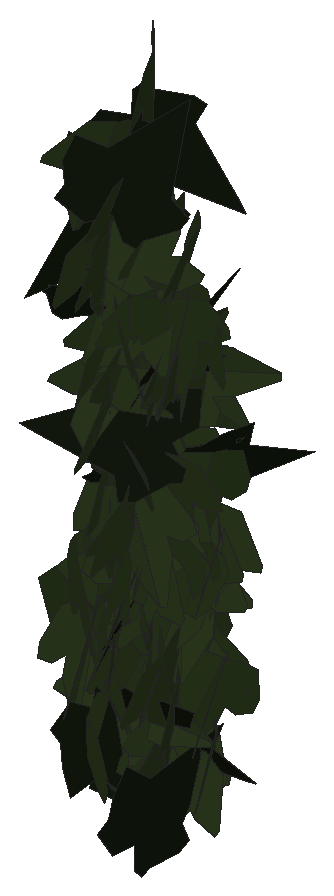
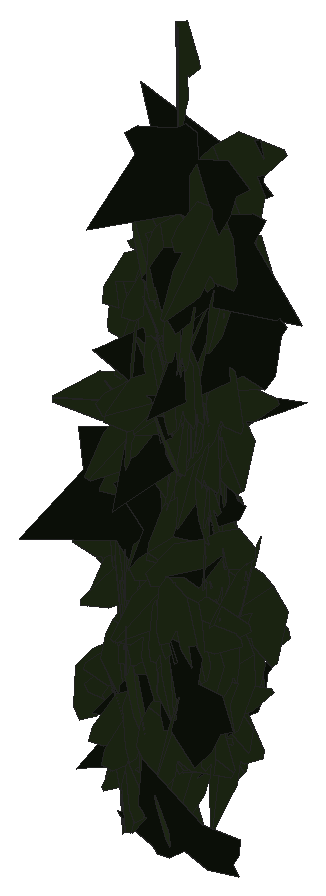
# SketchUp Ruby script. Lengths in inches.
U = 1.inch
M = Sketchup.active_model
def pt(a) = Geom::Point3d.new(a.map { |v| v * U })
def face(e, loops, mat)
  f = e.add_face(loops[0].map { |a| pt(a) })
  loops[1..].each { |l| e.add_face(l.map { |a| pt(a) }).erase! }
  f.material = f.back_material = mat if mat
  f
end
# faces: each face lists its corners as indices into pts; further lists are holes
def faces(e, pts, list, mat = nil) = list.each { |f| face(e, (f[0].is_a?(Array) ? f : [f]).map { |l| l.map { |i| pts[i] } }, mat) }
# xy, xz, yz: faces in a plane at the given z, y or x. An outline is a flat list of corners, or four numbers for a rectangle; further outlines are holes
def ring(l) = l.size == 4 ? [[l[0], l[1]], [l[2], l[1]], [l[2], l[3]], [l[0], l[3]]] : l.each_slice(2).to_a
def flat(e, list, mat, &to3) = list.each { |f| face(e, (f[0].is_a?(Array) ? f : [f]).map { |l| ring(l).map { |u, v| to3.(u, v) } }, mat) }
def xy(e, z, list, mat = nil) = flat(e, list, mat) { |x, y| [x, y, z] }
def xz(e, y, list, mat = nil) = flat(e, list, mat) { |x, z| [x, y, z] }
def yz(e, x, list, mat = nil) = flat(e, list, mat) { |y, z| [x, y, z] }
def lines(e, pts, list) = list.each { |a, b| e.add_line(pt(pts[a]), pt(pts[b])) }
# prism: a flat outline (further loops are holes) pulled along v
def prism(e, loops, v, mat = nil)
  f = face(e, loops, mat); d = Geom::Vector3d.new(v.map { |x| x * U })
  f.pushpull(f.normal.samedirection?(d) ? d.length : -d.length)
end
def box(e, o, s, mat = nil) = prism(e, [[o, [o[0] + s[0], o[1], o[2]], [o[0] + s[0], o[1] + s[1], o[2]], [o[0], o[1] + s[1], o[2]]]], [0, 0, s[2]], mat)
def at(x, y, z, deg = 0) = Geom::Transformation.translation(pt([x, y, z])) * Geom::Transformation.rotation(ORIGIN, Z_AXIS, deg.degrees)
def axes(o, x, y, z) = Geom::Transformation.new([*x, 0, *y, 0, *z, 0, *pt(o).to_a, 1])
def part(name) = M.definitions.add(name)
# library, detail: a bought-in or finely detailed component or shape, given as its bounding box
def library(name, o, s) = part(name).tap { |d| box(d.entities, o, s) }
def detail(e, o, s) = box(e.add_group.entities, o, s)
def put(e, d, t, mat = nil) = e.add_instance(d, t).tap { |i| i.material = mat if mat }
def group(e, t, mat = nil) = e.add_group.tap { |g| g.transformation = t; g.material = mat if mat }.entities
root = M.entities
M.materials.add("efeu1").color = [18, 25, 13]
M.materials.add("efeu2").color = [43, 57, 29]
c1 = part("ivyleaf_10")
p = [[0,0.5,-0.03],[-0.0625,2.02,-0.43],[-0.19,2.01,-0.46],[-0.54,1.05,-0.29],[-0.52,0.625,-0.18],[-0.83,0.76,-0.28],
  [-1.16,0.64,-0.33],[-1.15,0.33,-0.24],[-0.77,-0.39,0.02],[-0.3,-0.51,0.16],[0.04,-0.48,0.23],[-0.02,2.01,-0.4375],
  [-0.06,2.01,-0.43],[0.04,-0.49,0.23],[0.67,-0.49,0.14],[1.38,0.36,-0.2],[1.375,0.51,-0.24],[0.81,0.65,-0.19],
  [0.62,0.59,-0.15],[0.6,1.09,-0.28],[0.5,1.23,-0.31]]
faces(c1.entities,p,[[0,1,2,3,4,5,6,7,8,9,10],[11,12,0,13,14,15,16,17,18,19,20]],"efeu2")
c2 = part("ivyleaf_9")
p = [[1.54,2.16,1.25],[1.36,2.04,1.19],[-0.21,0.99,0.68],[-0.71,1.11,0.82],[-0.85,0.86,0.67],[-0.8,0.17,0.21],
  [-0.9,-0.01,0.1],[-0.67,-0.16,-0.02],[-0.08,-0.08,-0.05],[-0.03,-0.6,-0.4],[0.65,-0.88,-0.66],[0.83,-0.6,-0.49],
  [1.29,-0.42,-0.43],[1.8125,-0.07,-0.26],[1.21,0.44,0.15]]
faces(c2.entities,p,[[0,1,2,3,4,5,6,7,8,9,10,11,12,13,14]],"efeu1")
put(root,c1,axes([22.6875,224.7,214.85],[0.03755,-0.45322,-0.20781],[0.02712,0.20995,-0.45298],[0.49785,0.02275,0.04035]))
put(root,c1,axes([22.68,225.04,220.85],[-0.06561,-0.31766,-0.38051],[0.06416,0.37516,-0.32425],[0.49151,-0.09137,-0.00847]))
put(root,c1,axes([22.625,224.47,216.64],[-0.12805,0.47925,-0.06261],[0.01255,-0.06145,-0.49605],[-0.48316,-0.12861,0.00371]))
put(root,c1,axes([22.62,225.15,217.17],[0.2593,0.42528,-0.04357],[-0.02338,-0.03677,-0.4981],[-0.42687,0.26035,0.00082]))
put(root,c2,axes([22.86,224.98,220.58],[-0.04237,0.13988,-0.47816],[-0.02365,-0.47991,-0.1383],[-0.49764,0.01089,0.04728]))
put(root,c1,axes([22.73,224.58,215.93],[-0.17611,0.39993,-0.24299],[-0.09749,-0.28528,-0.39889],[-0.45769,-0.09312,0.17846]))
put(root,c1,axes([22.8125,224.86,218.66],[-0.27515,-0.37614,0.18114],[-0.04696,-0.18768,-0.46105],[0.41483,-0.27073,0.06795]))
put(root,c2,axes([22.71,225.38,213.77],[-0.41978,0.11401,0.24655],[0.23878,-0.06145,0.43498],[0.12949,0.48293,-0.00285]))
put(root,c1,axes([22.78,225.24,216.72],[-0.05871,-0.49513,0.03748],[-0.00529,-0.03711,-0.49859],[0.49651,-0.05894,-0.00088]))
put(root,c1,axes([22.86,225.27,216.29],[-0.36011,-0.31008,0.15546],[-0.09856,-0.12339,-0.47441],[0.33258,-0.37232,0.02774]))
put(root,c1,axes([22.78,224.65,221.42],[-0.12903,-0.4572,0.15595],[-0.00367,-0.16049,-0.47353],[0.48305,-0.12335,0.03806]))
put(root,c2,axes([22.57,224.55,219.71],[0.41909,0.25918,0.0848],[0.06905,0.04955,-0.49272],[-0.26381,0.4247,0.00574]))
put(root,c1,axes([22.77,224.91,219.05],[-0.48868,0.10307,-0.02389],[0.02379,-0.00294,-0.49942],[-0.10309,-0.48925,-0.00203]))
put(root,c1,axes([22.79,224.9,215.09],[-0.2091,-0.37415,0.25747],[0.05261,-0.30149,-0.39539],[0.45112,-0.13826,0.16545]))
put(root,c1,axes([22.75,224.46,220.32],[-0.01591,-0.43719,-0.2421],[0.08308,0.23653,-0.43261],[0.49279,-0.05399,0.06511]))
put(root,c1,axes([22.72,224.55,215.9],[0.30488,0.3849,-0.09434],[-0.05987,-0.07292,-0.49102],[-0.39175,0.31069,0.00163]))
put(root,c1,axes([22.89,225.42,215.2],[-0.0647,-0.34983,0.35133],[-0.08214,-0.34185,-0.35551],[0.48894,-0.10372,-0.01323]))
put(root,c1,axes([22.55,224.45,216.36],[-0.36033,-0.01903,-0.34612],[0.34663,-0.01684,-0.35995],[0.00204,-0.49935,0.02533]))
put(root,c1,axes([22.8,224.73,217.67],[0.14279,-0.42704,-0.21736],[0.01533,0.23076,-0.4433],[0.47893,0.11994,0.07899]))
put(root,c1,axes([22.61,225.16,217.99],[0.10332,-0.27071,0.40748],[0.28349,-0.30628,-0.27537],[0.39869,0.28794,0.0902]))
put(root,c1,axes([22.91,225.31,216.3],[-0.38221,-0.32073,0.03236],[-0.01778,-0.02913,-0.49883],[0.32187,-0.38247,0.01086]))
put(root,c1,axes([22.85,225,218.37],[-0.45896,0.19836,-0.0037],[0.00135,-0.00622,-0.49996],[-0.19839,-0.45893,0.00518]))
put(root,c1,axes([22.86,224.57,219.16],[0.02583,-0.40557,-0.29129],[0.02986,0.29241,-0.40448],[0.49844,0.0035,0.03932]))
put(root,c1,axes([22.92,224.83,217.88],[0.31506,-0.35458,-0.15814],[-0.10861,0.11504,-0.47431],[0.37275,0.33323,-0.00454]))
put(root,c1,axes([22.62,224.59,215.66],[-0.27958,0.21403,-0.355],[0.28131,-0.21653,-0.3521],[-0.30446,-0.39662,0.00066]))
put(root,c1,axes([22.8,225.1,219.28],[0.3207,-0.38339,0.01257],[0.1001,0.06782,-0.48516],[0.37031,0.3137,0.12026]))
put(root,c1,axes([22.9375,224.45,218.49],[0.13648,-0.45371,-0.15976],[-0.02047,0.16044,-0.47312],[0.48058,0.13569,0.02522]))
put(root,c1,axes([22.95,224.83,219.25],[-0.41607,-0.27599,-0.02676],[0.02157,0.0159,-0.49928],[0.27644,-0.41663,-0.00132]))
put(root,c1,axes([22.9375,225.01,217.37],[-0.13005,-0.46452,-0.13155],[0.04299,0.12455,-0.48233],[0.48087,-0.13676,0.00754]))
put(root,c2,axes([22.56,225.4,215.74],[0.01543,-0.0039,-0.49975],[0.41582,0.27746,0.01067],[0.27724,-0.41593,0.01181]))
put(root,c1,axes([23.14,224.52,218.03],[-0.37486,0.17021,0.28374],[-0.27494,0.07832,-0.41021],[-0.18409,-0.46357,0.03488]))
put(root,c1,axes([22.98,225.26,216.34],[0.05158,-0.4815,-0.12451],[-0.00997,0.12415,-0.48424],[0.49723,0.05244,0.0032]))
put(root,c1,axes([22.97,224.37,220.4],[0.16693,-0.45223,-0.13276],[0.00027,0.14093,-0.47973],[0.47131,0.16009,0.0473]))
put(root,c1,axes([23,224.49,216.09],[0.26145,-0.33283,-0.26621],[-0.0576,0.28185,-0.40895],[0.42228,0.24451,0.10904]))
put(root,c1,axes([22.85,225.01,214.62],[0.19151,0.45262,0.09197],[0.03571,0.08476,-0.49147],[-0.46049,0.19481,0.00014]))
put(root,c1,axes([23,225.28,216.5],[-0.25697,-0.42425,-0.06308],[0.03797,0.05074,-0.49597],[0.42723,-0.25969,0.00614]))
put(root,c1,axes([22.84,225.23,216.95],[-0.15281,-0.30265,-0.36749],[0.25408,0.27455,-0.33176],[0.40261,-0.28814,0.06988]))
put(root,c1,axes([23.07,224.18,214.92],[-0.17796,0.40184,0.23843],[-0.11876,0.20787,-0.43896],[-0.45191,-0.21287,0.02146]))
put(root,c1,axes([23.05,225.04,216.46],[0.04266,-0.48287,0.12254],[0.01746,-0.12146,-0.48471],[0.49787,0.04563,0.00649]))
put(root,c1,axes([22.99,224.6,218.94],[0.19174,-0.4321,0.16286],[0.07881,-0.14313,-0.47255],[0.455,0.20688,0.01322]))
put(root,c1,axes([23.05,224.47,220.99],[0.1837,-0.46417,0.02829],[0.00395,-0.02886,-0.49915],[0.46501,0.18361,-0.00694]))
put(root,c1,axes([22.93,225.26,215.32],[-0.17641,0.35657,-0.30288],[0.08652,-0.29325,-0.39563],[-0.45977,-0.192,0.04176]))
put(root,c1,axes([22.89,224.65,218.85],[0.00799,-0.16066,-0.47342],[0.24573,0.4136,-0.13622],[0.43538,-0.23049,0.08557]))
put(root,c1,axes([23.11,225.15,217.01],[-0.20633,-0.45518,0.01535],[0.00981,-0.02129,-0.49945],[0.45534,-0.2058,0.01772]))
put(root,c1,axes([23.04,225.12,219.1875],[-0.44355,0.21993,-0.06999],[0.03266,-0.09029,-0.49069],[-0.22847,-0.43986,0.06573]))
put(root,c2,axes([23.1875,224.71,216.33],[-0.27267,0.34544,-0.23732],[0.15223,-0.18216,-0.44005],[-0.39048,-0.31223,-0.00583]))
put(root,c1,axes([23.1,224.92,219.76],[0.08329,-0.49045,-0.05019],[0.00176,0.0512,-0.49737],[0.49301,0.08268,0.01025]))
put(root,c1,axes([23.06,224.98,219.77],[-0.39196,0.30905,-0.02924],[0.00924,-0.03546,-0.49866],[-0.31029,-0.39145,0.02209]))
put(root,c2,axes([22.94,224.28,215.09],[0.1653,-0.30794,-0.35756],[-0.14389,0.32792,-0.34894],[0.44941,0.21826,0.01979]))
put(root,c1,axes([23.1,224.91,219],[0.0593,-0.49138,0.07089],[0.01317,-0.06982,-0.49493],[0.4963,0.06057,0.00466]))
put(root,c1,axes([23.13,225.03,218.41],[-0.41126,0.27313,0.07914],[-0.07814,0.02525,-0.49321],[-0.27342,-0.41804,0.02192]))
put(root,c1,axes([23.1,224.38,216.86],[0.41223,-0.25881,-0.1144],[-0.0673,0.10668,-0.48383],[0.27485,0.41429,0.05312]))
put(root,c1,axes([22.82,224.82,216.56],[-0.16915,0.15078,-0.44571],[0.29807,-0.33213,-0.22548],[-0.36406,-0.34198,0.02247]))
put(root,c2,axes([22.75,224.96,217.36],[0.29717,0.3624,-0.17423],[0.11336,0.13235,0.46865],[0.3858,-0.31803,-0.0035]))
put(root,c1,axes([22.98,225.42,214.48],[0.22862,-0.37579,0.23773],[0.16194,-0.17859,-0.43804],[0.41413,0.27729,0.04005]))
put(root,c1,axes([23.14,224.74,216.98],[0.3451,-0.35655,-0.06147],[-0.04229,0.04462,-0.49621],[0.35933,0.34768,0.00064]))
put(root,c1,axes([23.125,225.34,214.92],[-0.23891,-0.40973,-0.15825],[0.07624,0.13873,-0.47428],[0.43256,-0.25075,-0.00381]))
put(root,c1,axes([23.16,224.66,217.28],[0.02213,-0.49859,0.03028],[0.0063,-0.03003,-0.49906],[0.49947,0.02247,0.00496]))
put(root,c1,axes([23.11,224.55,219.54],[-0.2429,0.43616,0.02754],[-0.01489,0.02323,-0.49924],[-0.43678,-0.24335,0.0017]))
put(root,c1,axes([23.18,225.45,215.3125],[0.06375,-0.495,0.03012],[-0.0022,-0.03065,-0.49905],[0.49591,0.0635,-0.00609]))
put(root,c1,axes([23.21,225.32,214.56],[0.04274,-0.49254,0.07471],[-0.00524,-0.07542,-0.49425],[0.49814,0.04146,-0.01161]))
put(root,c1,axes([23.15,225.39,215.2],[-0.35993,-0.33491,-0.09102],[0.11229,0.0117,-0.48709],[0.32839,-0.37108,0.0668]))
put(root,c1,axes([23.33,224.52,219.77],[0.41675,-0.06072,-0.2695],[-0.26598,0.04361,-0.42113],[0.07464,0.49438,0.00405]))
put(root,c1,axes([23.24,225.11,218.48],[-0.11445,-0.48033,0.07862],[0.00018,-0.08081,-0.49343],[0.48672,-0.11292,0.01867]))
put(root,c2,axes([22.92,224.95,221.59],[-0.03971,-0.0738,-0.49293],[0.24799,0.42601,-0.08376],[0.43234,-0.25114,0.00278]))
put(root,c2,axes([23.54,224.65,218.25],[-0.23768,-0.0335,0.43862],[-0.42843,-0.09546,-0.23945],[0.09978,-0.48966,0.01667]))
put(root,c1,axes([23.24,225.09,218.74],[0.06594,-0.13914,0.4757],[-0.13309,0.4573,0.15221],[-0.47743,-0.14669,0.02327]))
put(root,c2,axes([23.17,224.76,218.63],[0.23381,0.41258,0.15848],[0.07635,0.13888,-0.47422],[-0.43532,0.24595,0.00194]))
put(root,c1,axes([23.26,224.97,220.46],[0.06366,-0.49453,-0.0373],[0.00292,0.03798,-0.49855],[0.49592,0.06326,0.00772]))
put(root,c1,axes([23.5,224.74,217.03],[-0.38792,-0.0572,0.31024],[-0.29177,-0.12192,-0.38731],[0.11995,-0.48152,0.06121]))
put(root,c1,axes([23.23,224.35,216.19],[0.18528,-0.42221,0.19342],[-0.07231,0.17948,0.46104],[-0.45874,-0.19882,0.00545]))
put(root,c1,axes([23.32,225.09,214.74],[0.10039,-0.48179,-0.08834],[-0.02687,0.08462,-0.49205],[0.48908,0.10355,-0.0089]))
put(root,c1,axes([23.41,224.6,219.88],[-0.47335,-0.09411,0.13071],[-0.12129,-0.0587,-0.4815],[0.10597,-0.48754,0.03274]))
put(root,c1,axes([23.64,224.97,216.99],[-0.15636,-0.00653,0.47488],[-0.44928,-0.16002,-0.15013],[0.15394,-0.47366,0.04417]))
put(root,c1,axes([23.25,225.01,215.55],[0.33038,0.35808,-0.11236],[-0.07178,-0.08664,-0.48718],[-0.36837,0.33804,-0.00584]))
put(root,c1,axes([23.31,225.08,215.71],[0.24161,-0.37897,-0.21911],[-0.00709,0.24684,-0.43476],[0.43769,0.21319,0.11391]))
put(root,c1,axes([23.06,224.35,218.62],[0.21266,0.2354,0.38647],[0.21482,0.32332,-0.31514],[-0.39828,0.30008,0.03638]))
put(root,c1,axes([23.31,224.29,217.52],[0.03821,-0.43496,-0.24361],[0.04066,0.24623,-0.43326],[0.49688,0.0133,0.05419]))
put(root,c1,axes([23.33,225.08,217.92],[-0.37299,-0.33261,0.01569],[0.05856,-0.08871,-0.48857],[0.32779,-0.36263,0.10513]))
put(root,c1,axes([23.26,224.63,215.73],[-0.3389,-0.30215,-0.20941],[0.15483,0.14101,-0.45403],[0.33342,-0.37259,-0.00201]))
put(root,c1,axes([23.46,224.54,215.81],[0.24025,-0.32715,-0.29198],[-0.17717,0.23213,-0.40587],[0.40111,0.29848,-0.00438]))
put(root,c1,axes([23.35,225.31,215.64],[0.161,-0.46581,0.08424],[0.01085,-0.08533,-0.49255],[0.47324,0.16043,-0.01737]))
put(root,c2,axes([23.16,224.32,220.92],[-0.2702,0.03005,0.41963],[0.4109,-0.08819,0.27089],[0.0903,0.49124,0.02296]))
put(root,c2,axes([23.33,224.69,218.89],[-0.13464,0.43676,-0.20277],[-0.11772,0.17431,0.45361],[0.46692,0.16989,0.05589]))
put(root,c1,axes([23.35,224.48,216.81],[0.48947,-0.01147,-0.10144],[-0.10011,0.04335,-0.48795],[0.01999,0.49799,0.04014]))
put(root,c1,axes([23.1,225.14,218.17],[0.24502,-0.28203,-0.3323],[0.22736,-0.24252,0.37348],[-0.37185,-0.33413,0.0094]))
put(root,c1,axes([23.26,225.26,215.62],[0.46955,0.14588,0.09077],[0.02735,0.19732,-0.4586],[-0.16962,0.43564,0.17732]))
put(root,c1,axes([23.41,224.55,222.59],[0.20331,-0.40886,-0.20371],[-0.02157,0.21413,-0.45131],[0.45629,0.1923,0.06943]))
put(root,c1,axes([23.25,225.15,218.67],[-0.26249,-0.25424,-0.34127],[0.26403,0.21716,-0.36486],[0.33375,-0.37176,0.02025]))
put(root,c1,axes([23.37,224.96,214.54],[0.24288,0.40267,-0.16991],[-0.08539,-0.14692,-0.47024],[-0.42863,0.25743,-0.0026]))
put(root,c1,axes([23.5,225.27,216.625],[0.12433,-0.34536,-0.33951],[-0.10571,0.32272,-0.36699],[0.47262,0.16303,0.00723]))
put(root,c1,axes([23.3125,225.2,215.42],[0.45812,0.19747,0.03368],[-0.00226,0.08916,-0.49198],[-0.20031,0.45062,0.08258]))
put(root,c1,axes([23.03,224.53,215.13],[0.09459,0.04679,0.48874],[0.42626,0.23916,-0.10539],[-0.24364,0.43659,0.00535]))
put(root,c1,axes([23.23,224.51,220.22],[0.46112,0.09875,-0.16618],[0.16306,0.03217,0.47157],[0.10382,-0.4891,-0.00254]))
put(root,c1,axes([23.29,225.31,215.52],[0.20483,-0.38213,0.24904],[0.17571,-0.18582,-0.42965],[0.42091,0.26353,0.05817]))
put(root,c2,axes([23.1,224.63,214.95],[0.46517,0.05402,0.17522],[0.17436,0.01751,-0.46829],[-0.05673,0.49676,-0.00255]))
put(root,c1,axes([23.31,224.49,217.48],[-0.46026,-0.06932,-0.18264],[0.19526,-0.17718,-0.42483],[-0.00582,-0.46239,0.19017]))
put(root,c1,axes([23.36,224.91,215.99],[-0.04016,0.36824,-0.33584],[-0.0014,-0.33701,-0.36936],[-0.49838,-0.02872,0.0281]))
put(root,c1,axes([23.43,224.79,219.21],[0.24352,-0.43668,0.00304],[0.01229,0.00338,-0.49984],[0.43652,0.24351,0.01238]))
put(root,c1,axes([23.52,224.72,217.9],[-0.49729,-0.01165,0.05062],[-0.05054,-0.00416,-0.49742],[0.01201,-0.49985,0.00296]))
put(root,c1,axes([23.49,224.95,214.72],[0.2162,0.34433,-0.29102],[-0.16713,-0.23854,-0.40641],[-0.41872,0.27301,0.01195]))
put(root,c1,axes([23.49,224.64,214.625],[0.09293,-0.4906,-0.02598],[-0.00077,0.02629,-0.49931],[0.49129,0.09285,0.00413]))
put(root,c1,axes([23.46,224.6,219.8125],[-0.23042,-0.42466,-0.12874],[0.08145,0.10212,-0.48264],[0.4362,-0.24339,0.02212]))
put(root,c1,axes([23.61,224.9,214.42],[0.42429,0.00166,-0.26453],[-0.26448,0.01313,-0.42412],[0.00554,0.49982,0.01202]))
put(root,c1,axes([23.55,225.19,215.91],[-0.08764,-0.32387,0.37071],[-0.02765,-0.37271,-0.33215],[0.49148,-0.07872,0.04741]))
put(root,c1,axes([23.69,224.89,216.84],[-0.22749,-0.16945,0.41175],[-0.1649,-0.39744,-0.25466],[0.41359,-0.25166,0.12494]))
put(root,c1,axes([23.58,224.95,219.21],[0.1325,-0.44117,-0.19446],[-0.00246,0.20105,-0.45779],[0.48212,0.12227,0.05111]))
put(root,c1,axes([23.68,225.24,216.87],[0.18698,-0.345,-0.30986],[-0.12873,0.28235,-0.39206],[0.4455,0.22639,0.01676]))
put(root,c1,axes([23.44,225.28,216.76],[0.48813,-0.03621,0.10209],[0.10202,-0.00471,-0.48946],[0.0364,0.49867,0.00279]))
put(root,c1,axes([23.6,224.88,219.23],[-0.01677,-0.46093,-0.19304],[0.0475,0.19081,-0.45971],[0.49746,-0.03375,0.03739]))
put(root,c1,axes([23.52,224.96,216.47],[0.31106,0.39078,-0.02297],[-0.01565,-0.0169,-0.49947],[-0.39115,0.31145,0.00172]))
put(root,c1,axes([23.29,225.16,218.73],[-0.00846,-0.02587,0.49926],[0.33886,0.36683,0.02475],[-0.36756,0.33878,0.01133]))
put(root,c1,axes([23.63,224.48,215.76],[0.01831,-0.464,-0.18538],[0.02707,0.18615,-0.46327],[0.49893,0.00693,0.03193]))
put(root,c1,axes([23.64,224.93,216.65],[0.24615,0.39533,-0.182],[-0.15218,-0.11771,-0.4615],[-0.40774,0.28259,0.06237]))
put(root,c1,axes([23.65,224.625,215.38],[0.26109,-0.40347,-0.138],[-0.01894,0.15068,-0.47638],[0.426,0.25398,0.0634]))
put(root,c1,axes([23.64,225.34,215.34],[0.29891,-0.40078,-0.00579],[-0.00862,0.0008,-0.49993],[0.40072,0.29896,-0.00643]))
put(root,c1,axes([23.56,224.83,219.54],[0.3322,-0.34707,0.13853],[0.09071,-0.10491,-0.48038],[0.36251,0.3443,-0.00674]))
put(root,c1,axes([23.78,225.14,215.4375],[-0.32205,-0.32744,0.19765],[-0.10513,-0.17264,-0.45732],[0.36773,-0.33612,0.04235]))
put(root,c1,axes([23.72,225.14,214.66],[0.21478,-0.36479,-0.26608],[-0.08531,0.25656,-0.4206],[0.44339,0.22607,0.04797]))
put(root,c1,axes([23.7,224.51,219.8125],[-0.43562,-0.24515,-0.01149],[0.01307,0.0002,-0.49983],[0.24508,-0.43577,0.00623]))
put(root,c1,axes([23.67,224.86,220.44],[0.22375,-0.44714,-0.00194],[-0.00134,0.0015,-0.5],[0.44714,0.22375,-0.00053]))
put(root,c1,axes([23.74,224.91,219.59],[0.43405,-0.1306,-0.21106],[-0.14733,0.2066,-0.43082],[0.19974,0.43619,0.14087]))
put(root,c1,axes([23.6,225.26,217.02],[0.49572,0.06434,-0.01087],[-0.01112,0.00122,-0.49987],[-0.0643,0.49584,0.00264]))
put(root,c2,axes([23.49,225.13,217.63],[0.26092,0.23311,0.35718],[0.23848,0.26741,-0.34874],[-0.35362,0.35235,0.02836]))
put(root,c1,axes([23.72,225.08,217.78],[-0.2081,-0.44584,0.08901],[0.00618,-0.10066,-0.48972],[0.4546,-0.20272,0.0474]))
put(root,c2,axes([23.6,224.14,213.93],[-0.04781,-0.03431,0.49653],[0.32347,0.37696,0.05719],[-0.37826,0.32669,-0.01385]))
